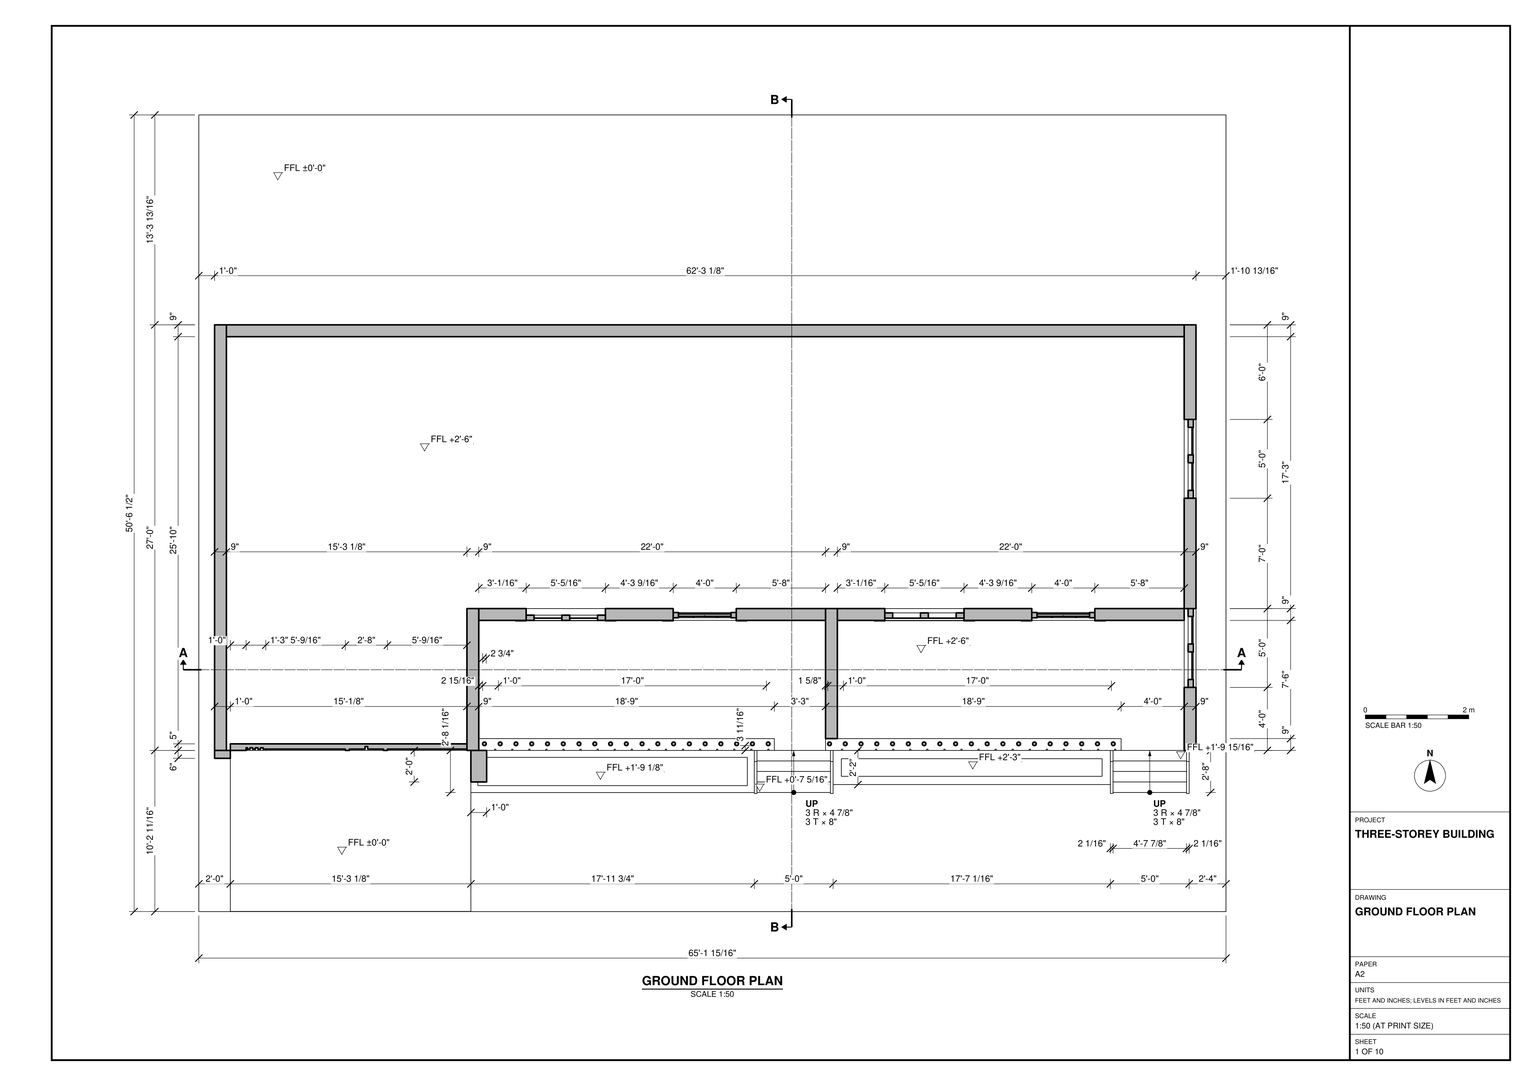
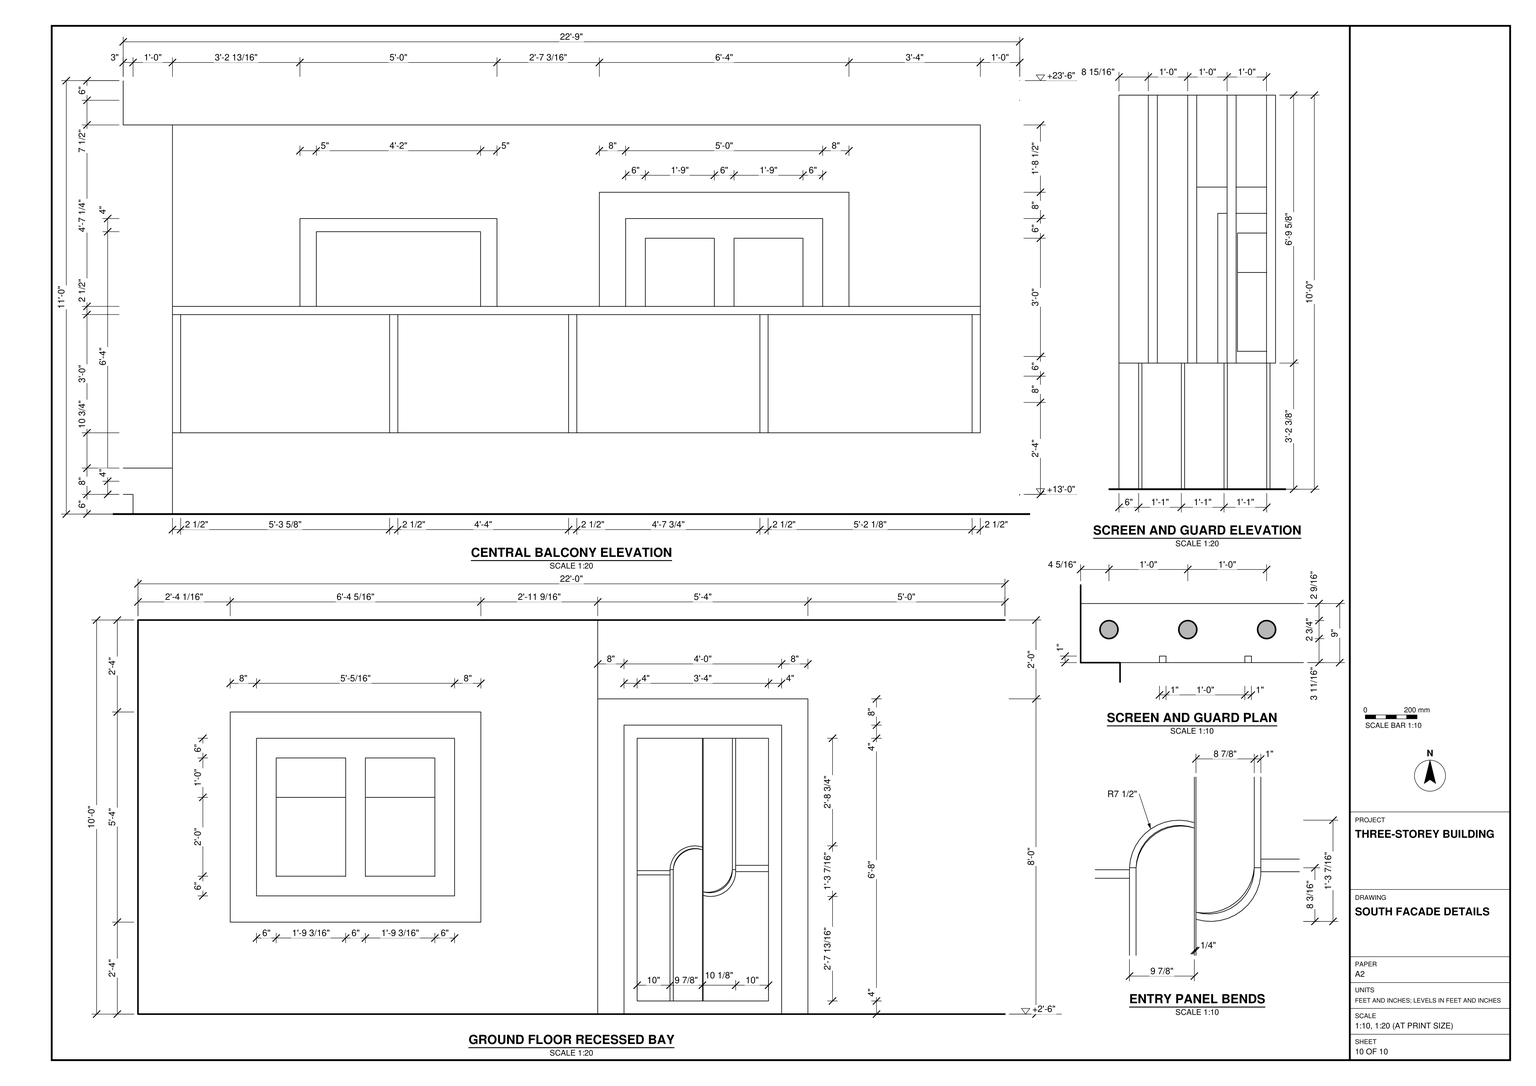
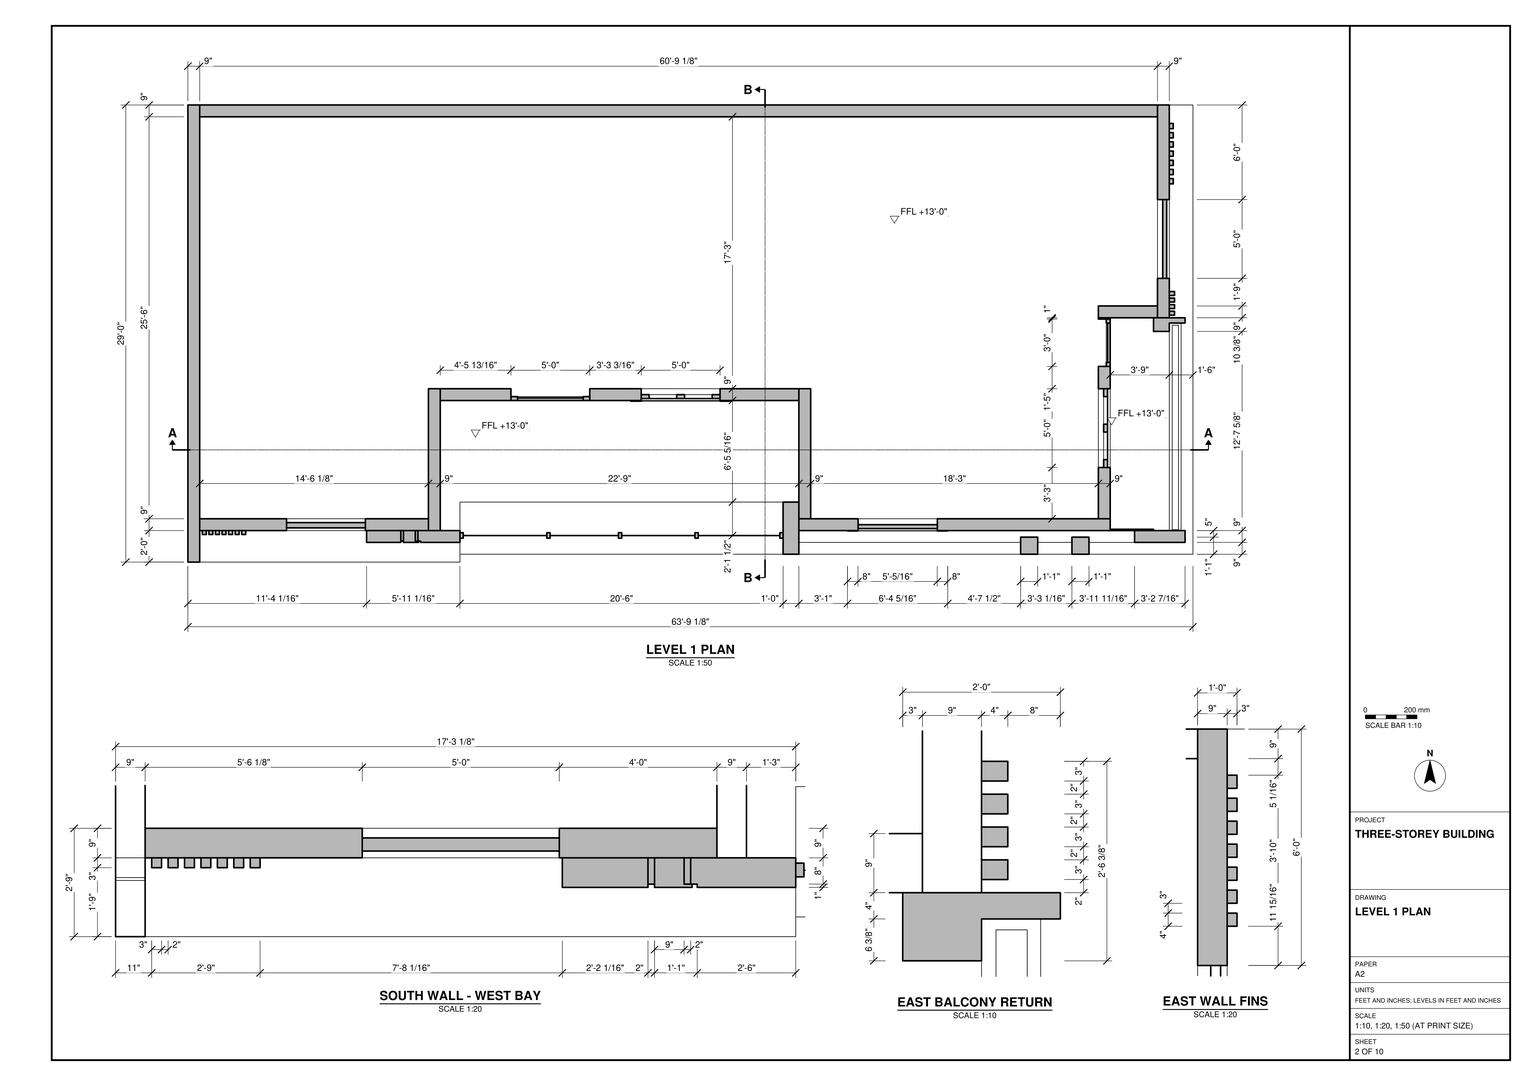
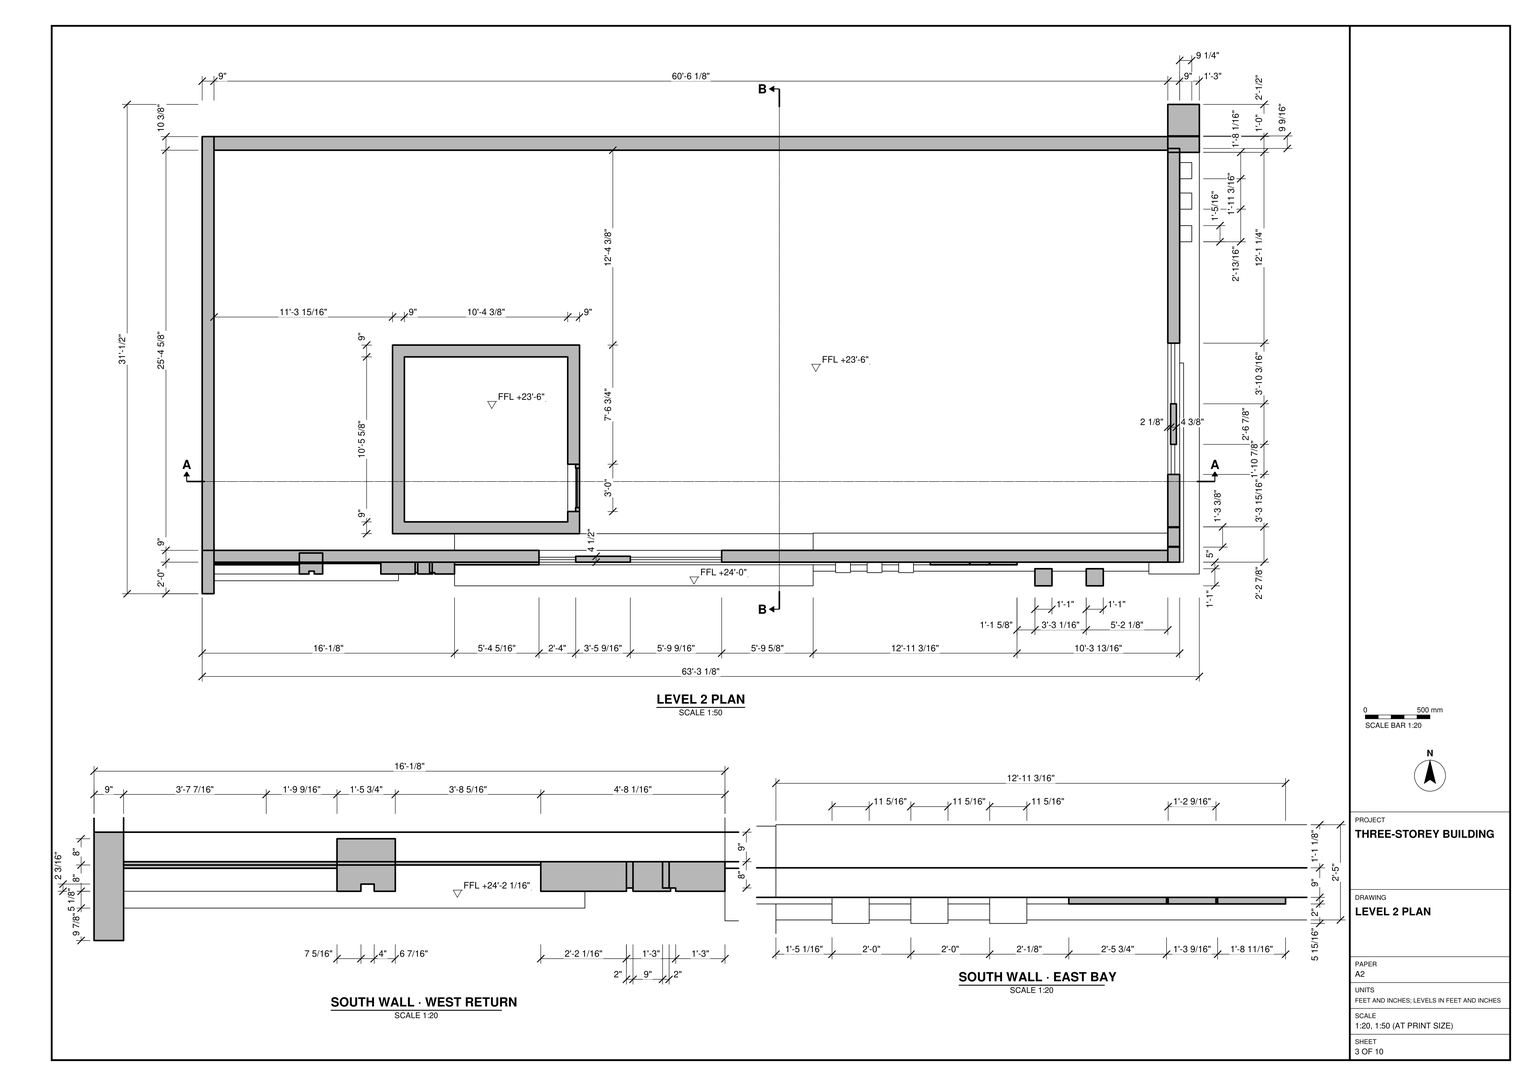
Build the three-storey building in SketchUp from task_files/diagram_01.pdf. Work in feet and inches. The overall model, including its base, is 65'-3 1/8" along x, 50'-6 1/2" along y and 35'-1 7/8" high. Use the levels ±0'-0", +13'-0" and +23'-6". Distinguish the ground datum from the raised ground-floor surface marked +2'-6".

Lay out each storey from its own plan. Model the walls at the thicknesses drawn, including the 9" perimeter walls, and follow the slab and roof outlines. On the south side, form the two recessed ground-floor bays with their dividing wall, framed windows, inset entry doors and short approach steps. Use the enlarged entry detail for the opposing bends in the door panels. Above these bays, set back the wall behind the central balcony and carry the guard across its front. Follow the details for the east balcony return, the wall fins and the screen above the guard. Place other openings, stairs, built-in joinery and main furniture where the sheets indicate them.

Keep walls, slabs, roof elements and each furniture or joinery piece in separate groups or components. Use components for repeated parts such as matching window units and fins. Decor and loose items, where shown, may be any suitable library components. Save one SketchUp model as output_files/three_storey_building_with_recessed_bays_and_balconies.skp.

# SketchUp Ruby script. Lengths in inches.
U = 1.inch
M = Sketchup.active_model
def pt(a) = Geom::Point3d.new(a.map { |v| v * U })
def face(e, loops, mat)
  f = e.add_face(loops[0].map { |a| pt(a) })
  loops[1..].each { |l| e.add_face(l.map { |a| pt(a) }).erase! }
  f.material = f.back_material = mat if mat
  f
end
# faces: each face lists its corners as indices into pts; further lists are holes
def faces(e, pts, list, mat = nil) = list.each { |f| face(e, (f[0].is_a?(Array) ? f : [f]).map { |l| l.map { |i| pts[i] } }, mat) }
# xy, xz, yz: faces in a plane at the given z, y or x. An outline is a flat list of corners, or four numbers for a rectangle; further outlines are holes
def ring(l) = l.size == 4 ? [[l[0], l[1]], [l[2], l[1]], [l[2], l[3]], [l[0], l[3]]] : l.each_slice(2).to_a
def flat(e, list, mat, &to3) = list.each { |f| face(e, (f[0].is_a?(Array) ? f : [f]).map { |l| ring(l).map { |u, v| to3.(u, v) } }, mat) }
def xy(e, z, list, mat = nil) = flat(e, list, mat) { |x, y| [x, y, z] }
def xz(e, y, list, mat = nil) = flat(e, list, mat) { |x, z| [x, y, z] }
def yz(e, x, list, mat = nil) = flat(e, list, mat) { |y, z| [x, y, z] }
def lines(e, pts, list) = list.each { |a, b| e.add_line(pt(pts[a]), pt(pts[b])) }
# prism: a flat outline (further loops are holes) pulled along v
def prism(e, loops, v, mat = nil)
  f = face(e, loops, mat); d = Geom::Vector3d.new(v.map { |x| x * U })
  f.pushpull(f.normal.samedirection?(d) ? d.length : -d.length)
end
def box(e, o, s, mat = nil) = prism(e, [[o, [o[0] + s[0], o[1], o[2]], [o[0] + s[0], o[1] + s[1], o[2]], [o[0], o[1] + s[1], o[2]]]], [0, 0, s[2]], mat)
def at(x, y, z, deg = 0) = Geom::Transformation.translation(pt([x, y, z])) * Geom::Transformation.rotation(ORIGIN, Z_AXIS, deg.degrees)
def axes(o, x, y, z) = Geom::Transformation.new([*x, 0, *y, 0, *z, 0, *pt(o).to_a, 1])
def part(name) = M.definitions.add(name)
# library, detail: a bought-in or finely detailed component or shape, given as its bounding box
def library(name, o, s) = part(name).tap { |d| box(d.entities, o, s) }
def detail(e, o, s) = box(e.add_group.entities, o, s)
def put(e, d, t, mat = nil) = e.add_instance(d, t).tap { |i| i.material = mat if mat }
def group(e, t, mat = nil) = e.add_group.tap { |g| g.transformation = t; g.material = mat if mat }.entities
root = M.entities
M.materials.add("[Color C01]").color = [209, 187, 166]
M.materials.add("[Color J01]").color = [112, 99, 124]
M.materials.add("[Color L11]").color = [109, 70, 75]
M.materials.add("[Color M00]").color = [255, 255, 255]
M.materials.add("[Color M02]").color = [198, 198, 198]
M.materials.add("[Color M05]").color = [114, 114, 114]
M.materials.add("[Color M07]").color = [58, 58, 58]
M.materials.add("[Color M08]").color = [30, 30, 30]
M.materials.add("[Color M09]").color = [0, 0, 0]
M.materials.add("[Concrete Stamped Ashlar]").color = [128, 71, 66]
M.materials.add("[Field Rectangle Tile]").color = [196, 189, 179]
M.materials.add("[Grass Dark Green]").color = [106, 157, 55]
M.materials.add("[Translucent Glass Gray]").color = [128, 128, 128]
M.materials["[Translucent Glass Gray]"].alpha = 0.5
M.materials.add("[Wood Bamboo]").color = [177, 105, 43]
M.materials.add("[Wood Cherry Original]").color = [152, 86, 42]
M.materials.add("[Wood Veneer 01]").color = [48, 28, 14]
c1 = part("Group\#20")
xz(c1.entities,0,[[0,0,21.16,36]])
c2 = part("Group\#21")
xz(c2.entities,0,[[0,0,21.16,36]])
c3 = part("Group\#41")
prism(c3.entities,[[[225,0,0],[221,0,0],[221,1,0],[220,1,0],[220,0,0],[208,0,0],[208,1,0],[207,1,0],[207,0,0],[195,0,0],[195,1,0],[194,1,0],[194,0,0],[182,0,0],[182,1,0],[181,1,0],[181,0,0],[169,0,0],[169,1,0],[168,1,0],[168,0,0],[156,0,0],[156,1,0],[155,1,0],[155,0,0],[143,0,0],[143,1,0],[142,1,0],[142,0,0],[130,0,0],[130,1,0],[129,1,0],[129,0,0],[117,0,0],[117,1,0],[116,1,0],[116,0,0],[104,0,0],[104,1,0],[103,1,0],[103,0,0],[91,0,0],[91,1,0],[90,1,0],[90,0,0],[78,0,0],[78,1,0],[77,1,0],[77,0,0],[65,0,0],[65,1,0],[64,1,0],[64,0,0],[52,0,0],[52,1,0],[51,1,0],[51,0,0],[39,0,0],[39,1,0],[38,1,0],[38,0,0],[26,0,0],[26,1,0],[25,1,0],[25,0,0],[13,0,0],[13,1,0],[12,1,0],[12,0,0],[0,0,0],[0,9,0],[225,9,0]]],[0,0,38.4])
c4 = library("Group\#42",[0,0,0],[60,32.82,59.54])
c5 = library("Group\#43",[0,0,0],[60,32.82,59.54])
c6 = part("Group\#52")
box(c6.entities,[0,0,0],[3,4,120])
c7 = part("Group\#127")
prism(c7.entities,[[[76.32,0.3,0],[0,0.3,0],[0,0.3,64],[76.32,0.3,64]],[[8,0.3,56],[8,0.3,8],[68.32,0.3,8],[68.32,0.3,56]]],[0,-0.3,0])
c8 = part("Group\#15")
prism(c8.entities,[[[64,0.3,0],[56,0.3,0],[56,0.3,88],[8,0.3,88],[8,0.3,0],[0,0.3,0],[0,0.3,96],[64,0.3,96]]],[0,-0.3,0])
p = [[8,0.3,0],[56,0.3,0]]
lines(c8.entities,p,[[0,1]])
c9 = library("Group\#23",[0,0,0],[48,4,88])
c10 = part("Group\#19")
prism(c10.entities,[[[0,0,48],[0,0,0],[60.32,0,0],[60.32,0,48]],[[33.16,0,42],[54.32,0,42],[54.32,0,6],[33.16,0,6]],[[27.16,0,42],[27.16,0,6],[6,0,6],[6,0,42]]],[0,4,0])
c11 = part("Group\#11")
prism(c11.entities,[[[0,78,4.5],[0,78,0.3],[0,70,0.3],[0,70,0],[0,68,0],[0,68,0.3],[0,60,0.3],[0,60,0],[0,58,0],[0,58,0.3],[0,50,0.3],[0,50,0],[0,48,0],[0,48,0.3],[0,40,0.3],[0,40,0],[0,38,0],[0,38,0.3],[0,30,0.3],[0,30,0],[0,28,0],[0,28,0.3],[0,20,0.3],[0,20,0],[0,18,0],[0,18,0.3],[0,10,0.3],[0,10,0],[0,8,0],[0,8,0.3],[0,0,0.3],[0,0,4.5],[0,8,4.5],[0,8,4],[0,10,4],[0,10,4.5],[0,18,4.5],[0,18,4],[0,20,4],[0,20,4.5],[0,28,4.5],[0,28,4],[0,30,4],[0,30,4.5],[0,38,4.5],[0,38,4],[0,40,4],[0,40,4.5],[0,48,4.5],[0,48,4],[0,50,4],[0,50,4.5],[0,58,4.5],[0,58,4],[0,60,4],[0,60,4.5],[0,68,4.5],[0,68,4],[0,70,4],[0,70,4.5]]],[30,0,0])
c12 = part("Group\#74")
box(c12.entities,[0,0,0],[4,3,120])
c13 = part("Group\#75")
box(c13.entities,[0,0,0],[4.75,2.9375,30])
c14 = part("Group\#83")
box(c14.entities,[0,0,0],[9.25,12.3125,20.4375])
c15 = part("Group\#84")
prism(c15.entities,[[[2.57,99.9375,2.0625],[2.7,99.9375,1.73],[2.75,99.9375,1.375],[2.7,99.9375,1.02],[2.57,99.9375,0.6875],[2.35,99.9375,0.4],[2.0625,99.9375,0.18],[1.73,99.9375,0.05],[1.375,99.9375,0],[1.02,99.9375,0.05],[0.6875,99.9375,0.18],[0.4,99.9375,0.4],[0.18,99.9375,0.6875],[0.05,99.9375,1.02],[0,99.9375,1.375],[0.05,99.9375,1.73],[0.18,99.9375,2.0625],[0.4,99.9375,2.35],[0.6875,99.9375,2.57],[1.02,99.9375,2.7],[1.375,99.9375,2.75],[1.73,99.9375,2.7],[2.0625,99.9375,2.57],[2.35,99.9375,2.35]]],[0,-99.9375,0])
c16 = library("Group\#86",[0,-2,0],[180.12,5,114])
c17 = part("Group\#91")
box(c17.entities,[0,0,0],[3,3,112])
c18 = part("Group\#94")
box(c18.entities,[0,0.625,-26.4],[12.98,13,201.25])
c19 = part("Group\#99")
box(c19.entities,[0,0,0],[2.5,4.1875,36])
c20 = part("Group\#110")
prism(c20.entities,[[[0,1.84,0.69],[0,1.75,0.47],[0,1.6,0.27],[0,1.41,0.125],[0,1.18,0.03],[0,0.9375,0],[0,0.69,0.03],[0,0.47,0.125],[0,0.27,0.27],[0,0.125,0.47],[0,0.03,0.69],[0,0,0.9375],[0,0.03,1.18],[0,0.125,1.41],[0,0.27,1.6],[0,0.47,1.75],[0,0.69,1.84],[0,0.9375,1.875],[0,1.18,1.84],[0,1.41,1.75],[0,1.6,1.6],[0,1.75,1.41],[0,1.84,1.18],[0,1.875,0.9375]]],[139.0625,0,0])
c21 = part("Group\#113")
prism(c21.entities,[[[64.98,1.52,0.41],[64.98,1.6,0.6],[64.98,1.625,0.8125],[64.98,1.6,1.02],[64.98,1.52,1.22],[64.98,1.39,1.39],[64.98,1.22,1.52],[64.98,1.02,1.6],[64.98,0.8125,1.625],[64.98,0.6,1.6],[64.98,0.41,1.52],[64.98,0.24,1.39],[64.98,0.11,1.22],[64.98,0.03,1.02],[64.98,0,0.8125],[64.98,0.03,0.6],[64.98,0.11,0.41],[64.98,0.24,0.24],[64.98,0.41,0.11],[64.98,0.6,0.03],[64.98,0.8125,0],[64.98,1.02,0.03],[64.98,1.22,0.11],[64.98,1.39,0.24]]],[-64.98,0,0])
c22 = part("Group\#129")
prism(c22.entities,[[[0.18,2.0625,0],[0.4,2.35,0],[0.6875,2.57,0],[1.02,2.7,0],[1.375,2.75,0],[1.73,2.7,0],[2.0625,2.57,0],[2.35,2.35,0],[2.57,2.0625,0],[2.7,1.73,0],[2.75,1.375,0],[2.7,1.02,0],[2.57,0.6875,0],[2.35,0.4,0],[2.0625,0.18,0],[1.73,0.05,0],[1.375,0,0],[1.02,0.05,0],[0.6875,0.18,0],[0.4,0.4,0],[0.18,0.6875,0],[0.05,1.02,0],[0,1.375,0],[0.05,1.73,0]]],[0,0,81.6])
xz(root,90.68,[[693.92,31.32,695.97,67.32]],"[Color M08]")
p = [[756.11,274.31,312],[756.11,434.68,312],[756.11,434.68,360]]
lines(root,p,[[0,1],[1,2]])
g1 = group(root,at(120,44.5,0))
box(g1,[-120,-44.5,0],[781.9375,606.5,24])
g2 = group(root,at(150.11,86.68,6))
box(g2,[-138.11,36,18],[738.11,324,30])
put(root,c1,at(282.36,223.38,84),"[Translucent Glass Gray]")
put(root,c2,at(255.2,223.38,84),"[Translucent Glass Gray]")
put(root,c3,at(477.11,122.68,54),"[Concrete Stamped Ashlar]")
put(root,c4,at(693.92,89.86,24))
put(root,c5,at(422.86,89.86,24))
put(root,c3,at(213.12,122.68,54),"[Concrete Stamped Ashlar]")
g3 = group(root,at(12,122.68,54))
box(g3,[0,0,0],[9,324,120])
g4 = group(root,at(207.12,110.68,24))
xy(g4,0,[[0,-12,12,12]])
xy(g4,156,[[-195.12,-12,-195.12,336,-186.12,336,-186.12,12,0,12,0,-12]])
xy(g4,164,[[-186.12,-12,12,12]])
xy(g4,282,[[-195.12,21,-186.12,336]])
xy(g4,388.875,[[-186.12,-12,-65.99,21]])
xy(g4,397.875,[[-195.12,-12,-65.99,21]])
xz(g4,-12,[[0,0,12,0,12,164,-186.12,164,-186.12,388.875,-65.99,388.875,-65.99,397.875,-195.12,397.875,-195.12,156,0,156]])
xz(g4,12,[[0,0,0,156,-186.12,156,-186.12,164,12,164,12,0]])
xz(g4,21,[[-195.12,282,-195.12,397.875,-65.99,397.875,-65.99,388.875,-186.12,388.875,-186.12,282]])
xz(g4,336,[[-195.12,156,-186.12,282]])
yz(g4,-195.12,[[-12,156,-12,397.875,21,397.875,21,282,336,282,336,156]])
yz(g4,-186.12,[[12,156,336,164],[-12,164,336,164,336,282,21,282,21,388.875,-12,388.875]])
yz(g4,-65.99,[[-12,388.875,21,397.875]])
yz(g4,0,[[-12,0,12,156]])
yz(g4,12,[[-12,0,12,164]])
g5 = group(root,at(12,116.68,24),"[Color J01]")
prism(g5,[[[0,0,0],[12,0,0],[12,0,144],[195.12,0,144],[195.12,0,156],[0,0,156]]],[0,6,0])
put(root,c6,at(759.11,428.64,180),"[Color L11]")
put(root,c6,at(759.11,421.64,180),"[Color L11]")
put(root,c6,at(759.11,414.64,180),"[Color L11]")
put(root,c6,at(759.11,407.64,180),"[Color L11]")
put(root,c6,at(759.11,400.64,180),"[Color L11]")
put(root,c6,at(759.11,393.64,180),"[Color L11]")
put(root,c6,at(759.11,386.64,180),"[Color L11]")
put(root,c1,at(555.36,223.38,96),"[Translucent Glass Gray]")
g6 = group(root,at(757.11,347.68,228),"[Translucent Glass Gray]")
yz(g6,0,[[0,0,21,36]])
g7 = group(root,at(754.11,314.68,222),"[Color M07]")
prism(g7,[[[3,60,48],[3,0,48],[3,0,0],[3,60,0]],[[3,33,6],[3,33,42],[3,54,42],[3,54,6]],[[3,6,42],[3,27,42],[3,27,6],[3,6,6]]],[-3,0,0])
g8 = group(root,at(756.11,347.68,96),"[Translucent Glass Gray]")
yz(g8,0,[[0,0,21,36]])
g9 = group(root,at(69.12,437.68,54))
box(g9,[-48.12,0,0],[729.11,9,120])
g10 = group(root,at(367.5,221.68,54),"[Color C01]")
xy(g10,0,[[118.62,0,266.61,9],[314.61,0,382.61,9]])
xy(g10,36,[[154.7,0,215.02,9]])
xy(g10,84,[[154.7,0,215.02,9]])
xy(g10,88,[[266.61,0,314.61,9]])
xy(g10,120,[[118.62,0,382.61,9]])
xz(g10,0,[[258.61,0,266.61,0,266.61,88,314.61,88,314.61,0,382.61,0,382.61,120,258.61,120]])
xz(g10,0,[[[118.62,0,258.61,120],[154.7,36,215.02,84]]],"[Field Rectangle Tile]")
xz(g10,9,[[[118.62,0,118.62,120,382.61,120,382.61,0,314.61,0,314.61,88,266.61,88,266.61,0],[154.7,36,215.02,84]]])
yz(g10,118.62,[[0,0,9,120]])
yz(g10,154.7,[[0,36,9,84]])
yz(g10,215.02,[[0,36,9,84]])
yz(g10,266.61,[[0,0,9,88]])
yz(g10,314.61,[[0,0,9,88]])
yz(g10,382.61,[[0,0,9,120]])
put(root,c7,at(514.2,221.38,82),"[Wood Veneer 01]")
put(root,c8,at(626.11,221.38,54),"[Wood Veneer 01]")
g11 = group(root,at(757.11,320.68,228),"[Translucent Glass Gray]")
yz(g11,0,[[0,0,21,36]])
g12 = group(root,at(756.11,320.68,96),"[Translucent Glass Gray]")
yz(g12,0,[[0,0,21,36]])
put(root,c9,at(634.11,223.68,54))
g13 = group(root,at(750.11,284.68,180),"[Color C01]")
prism(g13,[[[0,162,0],[0,0,0],[0,0,120],[0,162,120]],[[0,30,90],[0,30,42],[0,90,42],[0,90,90]]],[9,0,0])
g14 = group(root,at(204.12,122.68,174))
xy(g14,0,[[273,-18,273,0,-192.12,0,-192.12,324,572.99,324,572.99,-18]])
xy(g14,6,[[273,-18,572.99,-18,572.99,324,-192.12,324,-192.12,0,273,0]])
xz(g14,-18,[[273,0,572.99,6]],"[Color L11]")
xz(g14,0,[[-192.12,0,273,6]])
xz(g14,324,[[-192.12,0,572.99,6]])
yz(g14,-192.12,[[0,0,324,6]])
yz(g14,273,[[-18,0,0,6]])
yz(g14,572.99,[[-18,0,324,6]],"[Color L11]")
p = [[273,9,0],[273,9,6],[271.2,0,0]]
lines(g14,p,[[0,1],[1,2]])
put(root,c7,at(241.2,221.38,82),"[Wood Veneer 01]")
put(root,c9,at(361.11,223.68,54))
put(root,c8,at(353.11,221.38,54),"[Wood Veneer 01]")
g15 = group(root,at(94.5,221.68,54),"[Color C01]")
xy(g15,0,[[118.62,0,266.61,9],[314.61,0,382.61,9]],"[Field Rectangle Tile]")
xy(g15,36,[[154.7,0,215.02,9]],"[Field Rectangle Tile]")
xy(g15,84,[[154.7,0,215.02,9]],"[Field Rectangle Tile]")
xy(g15,88,[[266.61,0,314.61,9]],"[Field Rectangle Tile]")
xy(g15,120,[[118.62,0,382.61,9]],"[Field Rectangle Tile]")
xz(g15,0,[[258.61,0,266.61,0,266.61,88,314.61,88,314.61,0,382.61,0,382.61,120,258.61,120]])
xz(g15,0,[[[118.62,0,258.61,120],[154.7,36,215.02,84]]],"[Field Rectangle Tile]")
xz(g15,9,[[[118.62,0,118.62,120,382.61,120,382.61,0,314.61,0,314.61,88,266.61,88,266.61,0],[154.7,36,215.02,84]]],"[Field Rectangle Tile]")
yz(g15,118.62,[[0,0,9,120]],"[Field Rectangle Tile]")
yz(g15,154.7,[[0,36,9,84]],"[Field Rectangle Tile]")
yz(g15,215.02,[[0,36,9,84]],"[Field Rectangle Tile]")
yz(g15,266.61,[[0,0,9,88]],"[Field Rectangle Tile]")
yz(g15,314.61,[[0,0,9,88]],"[Field Rectangle Tile]")
yz(g15,382.61,[[0,0,9,120]],"[Field Rectangle Tile]")
g16 = group(root,at(204.12,122.68,54))
xy(g16,0,[[0,0,9,108]])
xy(g16,120,[[0,0,9,108]])
xz(g16,0,[[0,0,9,120]])
xz(g16,108,[[0,0,9,120]])
yz(g16,0,[[0,0,108,120]])
yz(g16,9,[[0,0,108,120]],"[Field Rectangle Tile]")
put(root,c10,at(249.2,221.68,90),"[Color M07]")
g17 = group(root,at(477.11,110.68,54))
xy(g17,0,[[0,21,9,120]])
xy(g17,120,[[0,21,9,120]])
xz(g17,21,[[0,0,9,120]])
xz(g17,120,[[0,0,9,120]])
yz(g17,0,[[21,0,120,120]])
yz(g17,9,[[21,0,120,120]],"[Field Rectangle Tile]")
put(root,c11,axes([759.11,305.68,138],[0.8,0,0],[0,1,0],[0,0,1]),"[Color L11]")
g18 = group(root,at(753.11,314.68,90),"[Color M07]")
prism(g18,[[[0,0,0],[0,0,48],[0,60,48],[0,60,0]],[[0,33,42],[0,33,6],[0,54,6],[0,54,42]],[[0,27,42],[0,6,42],[0,6,6],[0,27,6]]],[4,0,0])
g19 = group(root,at(750.11,98.68,18),"[Color C01]")
prism(g19,[[[9,24,6],[9,348,6],[9,348,156],[9,24,156]],[[9,132,120],[9,132,72],[9,72,72],[9,72,120]],[[9,216,72],[9,216,120],[9,276,120],[9,276,72]]],[-9,0,0])
put(root,c2,at(528.2,223.38,96),"[Translucent Glass Gray]")
put(root,c11,axes([759.11,305.68,269.97],[0.8,0,0],[0,1,0],[0,0,1]),"[Color L11]")
put(root,c10,at(522.2,223.38,90),"[Color M07]")
g20 = group(root,at(753.11,170.68,90),"[Color M07]")
prism(g20,[[[0,60,48],[0,60,0],[0,0,0],[0,0,48]],[[0,33,42],[0,33,6],[0,54,6],[0,54,42]],[[0,27,42],[0,6,42],[0,6,6],[0,27,6]]],[4,0,0])
g21 = group(root,at(756.11,176.68,96),"[Translucent Glass Gray]")
yz(g21,0,[[0,0,21,36]])
g22 = group(root,at(756.11,203.68,96),"[Translucent Glass Gray]")
yz(g22,0,[[0,0,21,36]])
g23 = group(root,at(759.11,161.68,138),"[Color L11]")
prism(g23,[[[0,78,4.5],[0,78,0.3],[0,70,0.3],[0,70,0],[0,68,0],[0,68,0.3],[0,60,0.3],[0,60,0],[0,58,0],[0,58,0.3],[0,50,0.3],[0,50,0],[0,48,0],[0,48,0.3],[0,40,0.3],[0,40,0],[0,38,0],[0,38,0.3],[0,30,0.3],[0,30,0],[0,28,0],[0,28,0.3],[0,20,0.3],[0,20,0],[0,18,0],[0,18,0.3],[0,10,0.3],[0,10,0],[0,8,0],[0,8,0.3],[0,0,0.3],[0,0,4.5],[0,8,4.5],[0,8,4],[0,10,4],[0,10,4.5],[0,18,4.5],[0,18,4],[0,20,4],[0,20,4.5],[0,28,4.5],[0,28,4],[0,30,4],[0,30,4.5],[0,38,4.5],[0,38,4],[0,40,4],[0,40,4.5],[0,48,4.5],[0,48,4],[0,50,4],[0,50,4.5],[0,58,4.5],[0,58,4],[0,60,4],[0,60,4.5],[0,68,4.5],[0,68,4],[0,70,4],[0,70,4.5]]],[24,0,0])
g24 = group(root,at(705.11,284.68,180))
box(g24,[0,0,0],[45,9,120])
g25 = group(root,at(705.11,176.68,180),"[Color C01]")
prism(g25,[[[0,71,0],[0,-45,0],[0,-45,120],[0,108,120],[0,108,0],[0,107,0],[0,107,89],[0,71,89]],[[0,-6,89],[0,-6,36],[0,54,36],[0,54,89]]],[9,0,0])
g26 = group(root,at(711.11,247.68,180),"[Wood Cherry Original]")
prism(g26,[[[3,36,0],[3,36,89],[3,0,89],[3,0,0]],[[3,33,3],[3,3,3],[3,3,86],[3,33,86]]],[-3,0,0])
g27 = group(root,at(712.11,250.68,183),"[Wood Cherry Original]")
box(g27,[0,0,0],[2,30,83])
g28 = group(root,at(477.11,122.68,180),"[Color J01]")
prism(g28,[[[237,9,0],[0,9,0],[0,9,120],[237,9,120]],[[105.41,9,90],[45.09,9,90],[45.09,9,42],[105.41,9,42]]],[0,-9,0])
g29 = group(root,at(709.11,170.68,216),"[Color M07]")
prism(g29,[[[0,0,0],[0,0,53],[0,60,53],[0,60,0]],[[0,33,47],[0,33,6],[0,54,6],[0,54,47]],[[0,27,47],[0,6,47],[0,6,6],[0,27,6]]],[3,0,0])
g30 = group(root,at(712.11,203.68,222),"[Translucent Glass Gray]")
yz(g30,0,[[0,0,21,41]])
g31 = group(root,at(712.11,176.68,222),"[Translucent Glass Gray]")
yz(g31,0,[[0,0,21,41]])
g32 = group(root,at(477.11,131.68,180))
box(g32,[0,0,0],[9,99,120])
g33 = group(root,at(29.87,221.68,180),"[Color C01]")
prism(g33,[[[447.24,9,0],[288.0625,9,0],[288.0625,9,84],[228.0625,9,84],[228.0625,9,0],[174.25,9,0],[174.25,9,120],[447.24,9,120]],[[387.24,9,84],[327.24,9,84],[327.24,9,36],[387.24,9,36]]],[0,-9,0])
g34 = group(root,at(195.12,122.68,180),"[Color C01]")
box(g34,[0,0,0],[9,108,120])
g35 = group(root,at(257.93,221.68,180))
g36 = group(g35,at(5,0,4),"[Wood Bamboo]")
box(g36,[0,0,0],[50,2,76])
g37 = group(g35,at(0,0,0),"[Wood Veneer 01]")
prism(g37,[[[60,3,84],[60,3,0],[0,3,0],[0,3,84]],[[55,3,4],[55,3,80],[5,3,80],[5,3,4]]],[0,-3,0])
g38 = group(root,at(357.11,223.18,216),"[Color M07]")
prism(g38,[[[0,3,48],[60,3,48],[60,3,0],[0,3,0]],[[27,3,6],[27,3,42],[6,3,42],[6,3,6]],[[54,3,42],[33,3,42],[33,3,6],[54,3,6]]],[0,-3,0])
g39 = group(root,at(390.11,223.18,222),"[Translucent Glass Gray]")
xz(g39,0,[[0,0,21,36]])
g40 = group(root,at(363.11,223.18,222),"[Translucent Glass Gray]")
xz(g40,0,[[0,0,21,36]])
g41 = group(root,at(349.11,221.18,208),"[Color L11]")
prism(g41,[[[0,0,0],[76,0,0],[76,0,64],[0,0,64]],[[8,0,56],[68,0,56],[68,0,8],[8,0,8]]],[0,0.5,0])
g42 = group(root,at(195.12,110.68,174))
xy(g42,0,[[24,-6,282,33.6875]])
xy(g42,6,[[282,3,575.99,12],[563.99,12,572.99,170],[551.99,163.625,551.99,174,575.99,174,575.99,170,563.99,170,563.99,163.625]])
xy(g42,18,[[563.99,12,572.99,170]])
xy(g42,24.75,[[24,-6,270,33.6875]])
xy(g42,44.375,[[282,3,537.56,12]])
xy(g42,102,[[563.99,12,575.99,170]])
xy(g42,118.5,[[9,-6,270,33.6875]],"[Color L11]")
xy(g42,126,[[551.99,174,575.99,336],[551.99,336,574.99,336.5],[551.99,336.5,575.99,360.5]])
xy(g42,138,[[9,-6,282,33.6875],[537.56,3,575.99,3,575.99,324,551.99,324,551.99,163.625,563.99,163.625,563.99,12,537.56,12]])
xy(g42,174,[[551.99,336,574.99,336.5]])
xy(g42,186,[[551.99,230.6875,575.99,324]])
xy(g42,195.25,[[551.99,230.6875,575.99,336],[551.99,336.5,575.99,360.5]])
xz(g42,-6,[[24,0,282,0,282,138,9,138,9,118.5,270,118.5,270,24.75,24,24.75]],"[Color L11]")
xz(g42,3,[[282,6,575.99,6,575.99,138,537.56,138,537.56,44.375,282,44.375]])
xz(g42,12,[[282,6,282,44.375,537.56,44.375,537.56,138,563.99,138,563.99,102,575.99,102,575.99,6,572.99,6,572.99,18,563.99,18,563.99,6],[563.99,6,572.99,18]])
xz(g42,33.6875,[[24,0,24,24.75,270,24.75,270,118.5,9,118.5,9,138,282,138,282,0]])
xz(g42,163.625,[[551.99,6,563.99,138]])
xz(g42,170,[[563.99,6,572.99,18],[572.99,6,575.99,6,575.99,102,563.99,102,563.99,18,572.99,18]])
xz(g42,174,[[551.99,6,575.99,126]])
xz(g42,230.6875,[[551.99,186,575.99,195.25]])
xz(g42,324,[[551.99,138,575.99,186]])
xz(g42,336,[[551.99,126,574.99,174],[574.99,126,575.99,174],[551.99,174,575.99,195.25]])
xz(g42,336.5,[[551.99,126,574.99,174],[574.99,126,575.99,174],[551.99,174,575.99,195.25]])
xz(g42,360.5,[[551.99,126,575.99,195.25]])
yz(g42,9,[[-6,118.5,33.6875,138]],"[Color L11]")
yz(g42,24,[[-6,0,33.6875,24.75]],"[Color L11]")
yz(g42,270,[[-6,24.75,33.6875,118.5]],"[Color L11]")
yz(g42,282,[[3,6,12,44.375],[12,6,33.6875,48]])
yz(g42,282,[[-6,0,33.6875,0,33.6875,6,3,6,3,44.375,12,44.375,12,48,33.6875,48,33.6875,138,-6,138]],"[Color L11]")
yz(g42,537.56,[[3,44.375,12,138]])
yz(g42,551.99,[[163.625,6,163.625,138,324,138,324,186,230.6875,186,230.6875,195.25,336,195.25,336,126,174,126,174,6],[336,126,336.5,174],[336.5,126,360.5,195.25]])
yz(g42,563.99,[[12,6,163.625,18],[163.625,6,170,18],[163.625,18,170,102],[12,102,163.625,138]])
yz(g42,572.99,[[12,6,170,18]],"[Color M07]")
yz(g42,574.99,[[336,126,336.5,174]])
yz(g42,575.99,[[3,6,12,6,12,102,170,102,170,6,174,6,174,126,336,126,336,195.25,230.6875,195.25,230.6875,186,324,186,324,138,3,138],[336.5,126,360.5,195.25]])
put(root,c12,at(759.11,286.68,180))
put(root,c12,at(759.11,291.68,180))
put(root,c12,at(759.11,296.68,180))
put(root,c12,at(759.11,301.68,180))
put(root,c13,at(761.3125,276.08,192),"[Color M09]")
put(root,c13,at(761.3125,217.77,192),"[Color M09]")
put(root,c13,at(761.3125,167.02,192),"[Color M09]")
put(root,c13,at(761.3125,123.4,192),"[Color M09]")
g43 = group(root,at(764.0625,220.71,192),"[Translucent Glass Gray]")
yz(g43,0,[[0,0,55.375,30]])
g44 = group(root,at(764.0625,169.96,192),"[Translucent Glass Gray]")
yz(g44,0,[[0,0,47.8125,30]])
g45 = group(root,at(764.0625,126.33,192),"[Translucent Glass Gray]")
yz(g45,0,[[0,0,40.6875,30]])
g46 = group(root,at(761.3125,123.4,222),"[Color M09]")
box(g46,[0,0,0],[4.75,155.625,1.4375])
g47 = group(root,at(12,437.68,180))
box(g47,[9,0,0],[729.11,9,120])
g48 = group(root,at(195.12,122.68,300))
prism(g48,[[[-174.12,0,0],[-174.12,324,0],[551.99,324,0],[551.99,151.625,0],[563.99,151.625,0],[563.99,0,0]]],[0,0,6])
g49 = group(root,at(747.11,122.68,306),"[Color C01]")
xy(g49,0,[[0,0,9,11.48],[0,11.48,9,11.98],[0,11.98,9,26.375],[0,26.375,9,26.875],[0,26.875,9,314.96]])
xy(g49,10.7,[[0,66.8,9,166.74]])
xy(g49,52.14,[[0,66.8,9,93.13]])
xy(g49,63.25,[[0,0,9,11.48],[0,11.48,9,11.98],[0,11.98,9,26.375],[0,26.375,9,26.875],[0,26.875,9,93.13],
  [0,166.74,9,314.96]])
xz(g49,0,[[0,0,9,63.25]])
xz(g49,11.48,[[0,0,9,63.25]])
xz(g49,11.98,[[0,0,9,63.25]])
xz(g49,26.375,[[0,0,9,63.25]])
xz(g49,26.875,[[0,0,9,63.25]])
xz(g49,66.8,[[0,10.7,9,52.14]])
xz(g49,93.13,[[0,52.14,9,63.25]])
xz(g49,166.74,[[0,10.7,9,63.25]])
xz(g49,314.96,[[0,0,9,63.25]])
yz(g49,0,[[0,0,11.48,63.25],[11.48,0,11.98,63.25],[11.98,0,26.375,63.25],[26.375,0,26.875,63.25],[26.875,0,26.875,63.25,93.13,63.25,93.13,52.14,66.8,52.14,66.8,10.7,166.74,10.7,166.74,63.25,314.96,63.25,314.96,0]])
yz(g49,9,[[0,0,11.48,63.25],[11.48,0,11.98,63.25],[11.98,0,26.375,63.25],[26.375,0,26.875,63.25],[26.875,0,314.96,0,314.96,63.25,166.74,63.25,166.74,10.7,66.8,10.7,66.8,52.14,93.13,52.14,93.13,63.25,26.875,63.25]])
put(root,c14,at(756.11,414.6,326.88),"[Color L11]")
put(root,c14,at(756.11,391.41,326.88),"[Color L11]")
put(root,c14,at(756.11,366.6,326.88),"[Color L11]")
put(root,c15,at(749.67,189.48,318.91),"[Color M09]")
put(root,c15,at(749.67,189.48,327.91),"[Color M09]")
put(root,c15,at(749.67,189.48,336.91),"[Color M09]")
put(root,c15,at(749.67,189.48,345.91),"[Color M09]")
put(root,c15,at(749.67,189.48,354.04),"[Color M09]")
put(root,c15,at(749.67,189.48,363.91),"[Color M09]")
g50 = group(root,at(749.23,212.375,316.26),"[Color L11]")
box(g50,[0,0,0],[4.4,30.875,59.74])
put(root,c16,at(24,124.68,54),"[Color M08]")
g51 = group(root,at(21,122.68,180),"[Color C01]")
prism(g51,[[[174.12,9,0],[0,9,0],[0,9,120],[174.12,9,120]],[[126.12,9,44],[126.12,9,92],[66.12,9,92],[66.12,9,44]]],[0,-9,0])
g52 = group(root,at(87.12,124.74,224),"[Color M07]")
prism(g52,[[[0,0,48],[0,0,0],[60,0,0],[60,0,48]],[[27,0,42],[27,0,6],[6,0,6],[6,0,42]],[[33,0,42],[54,0,42],[54,0,6],[33,0,6]]],[0,4,0])
g53 = group(root,at(120.12,124.74,230),"[Translucent Glass Gray]")
xz(g53,0,[[0,0,21,36]])
g54 = group(root,at(93.12,124.74,230),"[Translucent Glass Gray]")
xz(g54,0,[[0,0,21,36]])
g55 = group(root,at(77.77,122.18,272),"[Color L11]")
prism(g55,[[[70.6875,-0.25,4.5],[70.6875,-0.25,0.3],[70,-0.24,0.3],[70,-0.24,0],[68,-0.24,0],[68,-0.24,0.3],[60,-0.21,0.3],[60,-0.21,0],[58,-0.2,0],[58,-0.2,0.3],[50,-0.17,0.3],[50,-0.17,0],[48,-0.17,0],[48,-0.17,0.3],[40,-0.14,0.3],[40,-0.14,0],[38,-0.13,0],[38,-0.13,0.3],[30,-0.1,0.3],[30,-0.1,0],[28,-0.1,0],[28,-0.1,0.3],[20,-0.07,0.3],[20,-0.07,0],[18,-0.0625,0],[18,-0.0625,0.3],[10,-0.03,0.3],[10,-0.03,0],[8,-0.03,0],[8,-0.03,0.3],[0,0,0.3],[0,0,4.5],[8,-0.03,4.5],[8,-0.03,4],[10,-0.03,4],[10,-0.03,4.5],[18,-0.0625,4.5],[18,-0.0625,4],[20,-0.07,4],[20,-0.07,4.5],[28,-0.1,4.5],[28,-0.1,4],[30,-0.1,4],[30,-0.1,4.5],[38,-0.13,4.5],[38,-0.13,4],[40,-0.14,4],[40,-0.14,4.5],[48,-0.17,4.5],[48,-0.17,4],[50,-0.17,4],[50,-0.17,4.5],[58,-0.2,4.5],[58,-0.2,4],[60,-0.21,4],[60,-0.21,4.5],[68,-0.24,4.5],[68,-0.24,4],[70,-0.24,4],[70,-0.24,4.5]]],[-0.08,-24,0])
put(root,c17,at(23,119.68,188),"[Color L11]")
put(root,c17,at(28,119.68,188),"[Color L11]")
put(root,c17,at(33,119.68,188),"[Color L11]")
put(root,c17,at(38,119.68,188),"[Color L11]")
put(root,c17,at(43,119.68,188),"[Color L11]")
put(root,c17,at(48,119.68,188),"[Color L11]")
put(root,c17,at(53,119.68,188),"[Color L11]")
g56 = group(root,at(24,0.12,24),"[Color M00]")
prism(g56,[[[183.12,122.5625,0],[183.12,122.5625,30],[183.12,0,0]]],[-183.12,0,0],"[Color M00]")
g57 = group(root,at(12,115.46,154.17),"[Color M05]")
prism(g57,[[[0,1.22,3.4375],[195.12,0.875,3.4375],[195.12,0,3.4375],[0,0.35,3.4375]]],[0,0,22.39])
put(root,c18,at(684.99,104.06,206.4),"[Color L11]")
g58 = group(root,at(294.56,122.68,306),"[Color C01]")
prism(g58,[[[452.55,0,63.25],[112.91,0,63.25],[112.91,0,14.06],[-26.15,0,14.06],[-26.15,0,51.43],[8.26,0,51.43],[8.26,0,63.25],[-273.56,0,63.25],[-273.56,0,0],[452.55,0,0]]],[0,9,0])
g59 = group(root,at(714.11,122.68,206.4),"[Color C01]")
box(g59,[0,0,0],[33,1,86.04])
put(root,c18,at(645.93,104.06,206.4),"[Color L11]")
g60 = group(root,at(148.03,113.68,188),"[Color J01]")
xy(g60,0,[[0,0,26.08,9],[28.08,0,28.08,9,37.08,9,37.08,1,39.52,1,39.52,0],[41.08,0,41.08,1,39.08,1,39.08,9,71.08,9,71.08,0],[26.08,1,28.08,9],[37.08,1,39.08,9]])
xy(g60,112,[[56.08,0,71.08,9]])
xy(g60,181.25,[[0,0,26.08,9],[28.08,0,39.52,0,39.52,1,37.08,1,37.08,9,28.08,9],[41.08,0,56.08,0,56.08,9,39.08,9,39.08,1,41.08,1],[26.08,1,28.08,9],[37.08,1,39.08,9]])
xz(g60,0,[[0,0,26.08,181.25],[28.08,0,39.52,181.25],[41.08,0,71.08,0,71.08,112,56.08,112,56.08,181.25,41.08,181.25]])
xz(g60,1,[[26.08,0,28.08,181.25],[37.08,0,39.08,181.25],[39.08,0,39.52,181.25],[39.52,0,41.08,181.25]])
xz(g60,9,[[0,0,26.08,181.25],[26.08,0,28.08,181.25],[28.08,0,37.08,181.25],[37.08,0,39.08,181.25],[39.08,0,39.08,181.25,56.08,181.25,56.08,112,71.08,112,71.08,0]])
yz(g60,0,[[0,0,9,181.25]])
yz(g60,26.08,[[0,0,1,181.25],[1,0,9,181.25]])
yz(g60,28.08,[[0,0,1,181.25],[1,0,9,181.25]])
yz(g60,37.08,[[1,0,9,181.25]])
yz(g60,39.08,[[1,0,9,181.25]])
yz(g60,39.52,[[0,0,1,181.25]])
yz(g60,41.08,[[0,0,1,181.25]])
yz(g60,56.08,[[0,112,9,181.25]])
yz(g60,71.08,[[0,0,9,112]])
put(root,c19,at(219.12,116.89,198.75),"[Color M09]")
put(root,c19,at(285.24,116.89,198.75),"[Color M09]")
put(root,c19,at(339.74,116.89,198.75),"[Color M09]")
put(root,c19,at(397.99,116.89,198.75),"[Color M09]")
put(root,c19,at(462.61,116.89,198.75),"[Color M09]")
g61 = group(root,at(400.49,118.89,198.75),"[Translucent Glass Gray]")
xz(g61,0,[[0,0,62.12,36]])
g62 = group(root,at(342.24,118.89,198.75),"[Translucent Glass Gray]")
xz(g62,0,[[0,0,55.75,36]])
g63 = group(root,at(287.74,118.89,198.75),"[Translucent Glass Gray]")
xz(g63,0,[[0,0,52,36]])
g64 = group(root,at(221.62,118.89,198.75),"[Translucent Glass Gray]")
xz(g64,0,[[0,0,63.625,36]])
g65 = group(root,at(219.12,116.89,234.75),"[Color M09]")
box(g65,[0,0,0],[246,4.1875,2.5])
g66 = group(root,at(477.11,122.68,300))
box(g66,[0,-6.875,0],[270,29,6])
g67 = group(root,at(514.2,122.62,270.07),"[Color L11]")
prism(g67,[[[76.625,-0.27,4.5],[76.625,-0.27,0.3],[70,-0.24,0.3],[70,-0.24,0],[68,-0.24,0],[68,-0.24,0.3],[60,-0.21,0.3],[60,-0.21,0],[58,-0.2,0],[58,-0.2,0.3],[50,-0.17,0.3],[50,-0.17,0],[48,-0.17,0],[48,-0.17,0.3],[40,-0.14,0.3],[40,-0.14,0],[38,-0.13,0],[38,-0.13,0.3],[30,-0.1,0.3],[30,-0.1,0],[28,-0.1,0],[28,-0.1,0.3],[20,-0.07,0.3],[20,-0.07,0],[18,-0.0625,0],[18,-0.0625,0.3],[10,-0.03,0.3],[10,-0.03,0],[8,-0.03,0],[8,-0.03,0.3],[0,0,0.3],[0,0,4.5],[8,-0.03,4.5],[8,-0.03,4],[10,-0.03,4],[10,-0.03,4.5],[18,-0.0625,4.5],[18,-0.0625,4],[20,-0.07,4],[20,-0.07,4.5],[28,-0.1,4.5],[28,-0.1,4],[30,-0.1,4],[30,-0.1,4.5],[38,-0.13,4.5],[38,-0.13,4],[40,-0.14,4],[40,-0.14,4.5],[48,-0.17,4.5],[48,-0.17,4],[50,-0.17,4],[50,-0.17,4.5],[58,-0.2,4.5],[58,-0.2,4],[60,-0.21,4],[60,-0.21,4.5],[68,-0.24,4.5],[68,-0.24,4],[70,-0.24,4],[70,-0.24,4.5]]],[-0.08,-24,0])
g68 = group(root,at(522.2,124.18,222))
g69 = group(g68,at(6,0,6),"[Translucent Glass Gray]")
xz(g69,0,[[0,0,21.16,36]])
g70 = group(g68,at(0,0,0),"[Color M07]")
prism(g70,[[[60.32,3,48],[60.32,3,0],[0,3,0],[0,3,48]],[[27.16,3,6],[27.16,3,42],[6,3,42],[6,3,6]],[[54.32,3,42],[33.16,3,42],[33.16,3,6],[54.32,3,6]]],[0,-3,0])
g71 = group(g68,at(33.16,0,6),"[Translucent Glass Gray]")
xz(g71,0,[[0,0,21.16,36]])
g72 = group(root,at(204.12,120.68,313.75))
xy(g72,0,[[0,0,391.9375,2],[391.9375,0,392.4375,2],[392.4375,0,407,2],[407,0,407.5,2],[407.5,0,428.1875,2]])
xy(g72,10.04,[[64.29,0,362.1875,2]])
xy(g72,43.68,[[64.29,0,98.71,2]])
xy(g72,44.17,[[273,0,362.1875,2]])
xy(g72,55.5,[[0,0,98.71,2],[391.9375,0,392.4375,2],[392.4375,0,407,2],[407,0,407.5,2],[407.5,0,428.1875,2]])
xy(g72,59.625,[[273,0,391.9375,2]])
xz(g72,0,[[0,0,391.9375,0,391.9375,59.625,273,59.625,273,44.17,362.1875,44.17,362.1875,10.04,64.29,10.04,64.29,43.68,98.71,43.68,98.71,55.5,0,55.5],[391.9375,0,392.4375,55.5],[392.4375,0,407,55.5],[407,0,407.5,55.5],[407.5,0,428.1875,55.5]])
xz(g72,2,[[0,0,0,55.5,98.71,55.5,98.71,43.68,64.29,43.68,64.29,10.04,362.1875,10.04,362.1875,44.17,273,44.17,273,59.625,391.9375,59.625,391.9375,0],[391.9375,0,392.4375,55.5],[392.4375,0,407,55.5],[407,0,407.5,55.5],[407.5,0,428.1875,55.5]])
yz(g72,0,[[0,0,2,55.5]])
yz(g72,64.29,[[0,10.04,2,43.68]])
yz(g72,98.71,[[0,43.68,2,55.5]])
yz(g72,273,[[0,44.17,2,59.625]])
yz(g72,362.1875,[[0,10.04,2,44.17]])
yz(g72,391.9375,[[0,0,2,55.5],[0,55.5,2,59.625]])
yz(g72,392.4375,[[0,0,2,55.5]])
yz(g72,407,[[0,0,2,55.5]])
yz(g72,407.5,[[0,0,2,55.5]])
yz(g72,428.1875,[[0,0,2,55.5]])
g73 = group(root,at(542.21,108.74,334.21),"[Color L11]")
box(g73,[0,6,0],[11.3125,7.9375,14.9375])
g74 = group(root,at(518.21,108.74,334.21),"[Color L11]")
box(g74,[0,6,0],[11.3125,7.9375,14.9375])
g75 = group(root,at(494.21,108.74,334.21),"[Color L11]")
box(g75,[0,6,0],[11.3125,7.9375,14.9375])
g76 = group(root,at(296.39,122.68,323.79),"[Color L11]")
box(g76,[0,0,0],[41.56,4.5,57.46])
put(root,c20,at(268.41,124.57,322.89),"[Color M09]")
put(root,c20,at(268.41,124.57,330.89),"[Color M09]")
put(root,c20,at(268.41,124.57,338.89),"[Color M09]")
put(root,c20,at(268.41,124.57,346.89),"[Color M09]")
put(root,c20,at(268.41,124.57,354.14),"[Color M09]")
put(root,c20,at(268.41,124.57,362.89),"[Color M09]")
g77 = group(root,at(21,108.56,300),"[Color L11]")
box(g77,[0,0,0],[140.47,14.125,14.08])
g78 = group(root,at(85.98,113.68,314.08),"[Color J01]")
prism(g78,[[[0,16,0],[17.75,16,0],[17.75,0,0],[11.32,0,0],[11.32,2.1875,0],[7.29,2.1875,0],[7.29,0,0],[0,0,0]]],[0,0,98.8])
put(root,c21,at(21,125.57,371.63),"[Color M09]")
put(root,c21,at(21,125.57,377.63),"[Color M09]")
put(root,c21,at(21,125.57,383.63),"[Color M09]")
put(root,c21,at(21,125.57,389.63),"[Color M09]")
put(root,c21,at(21,125.57,395.63),"[Color M09]")
put(root,c21,at(21,125.57,401.63),"[Color M09]")
put(root,c21,at(21,125.57,407.63),"[Color M09]")
put(root,c21,at(21,125.57,413.63))
put(root,c21,at(21,125.57,419.63))
g79 = group(root,at(21,436.33,306))
box(g79,[0,0,0],[726.11,10.36,63.25])
g80 = group(root,at(12,131.68,306))
box(g80,[0,0,0],[9,315,63.25])
g81 = group(root,at(21,121.68,314.08),"[Color L11]")
box(g81,[0,0,0],[127.03,1,55.17])
g82 = group(root,at(21,113.68,348.58),"[Color J01]")
prism(g82,[[[64.98,8,0],[64.98,8,20.67],[64.98,0,20.67],[64.98,0,17.96],[64.98,7,17.96],[64.98,7,3.63],[64.98,0,3.63],[64.98,0,0]]],[-64.98,0,0])
g83 = group(root,at(21,113.68,314.08),"[Color J01]")
prism(g83,[[[43.43,8,0],[43.43,8,34.51],[43.43,0,34.51],[43.43,0,29.14],[43.43,7,29.14],[43.43,7,27.09],[43.43,0,27.09],[43.43,0,20.74],[43.43,7,20.74],[43.43,7,17.9],[43.43,0,17.9],[43.43,0,8.95],[43.43,7,8.95],[43.43,7,6.08],[43.43,0,6.08],[43.43,0,0]]],[-43.43,0,0])
g84 = group(root,at(156.93,144.37,306),"[Color C01]")
xy(g84,0,[[[0,0,142.36,143.6],[9,9,133.36,134.6]]])
xy(g84,3.32,[[133.36,16.875,142.36,52.875]])
xy(g84,84,[[133.36,16.875,142.36,52.875]])
xy(g84,94.875,[[[0,0,142.36,143.6],[9,9,133.36,134.6]]])
xz(g84,0,[[0,0,142.36,94.875]])
xz(g84,9,[[9,0,133.36,94.875]])
xz(g84,16.875,[[133.36,3.32,142.36,84]])
xz(g84,52.875,[[133.36,3.32,142.36,84]])
xz(g84,134.6,[[9,0,133.36,94.875]])
xz(g84,143.6,[[0,0,142.36,94.875]])
yz(g84,0,[[0,0,143.6,94.875]])
yz(g84,9,[[9,0,134.6,94.875]])
yz(g84,133.36,[[[9,0,134.6,94.875],[16.875,3.32,52.875,84]]])
yz(g84,142.36,[[[0,0,143.6,94.875],[16.875,3.32,52.875,84]]])
g85 = group(root,at(139.37,131.68,400.875),"[Color L11]")
box(g85,[9.3125,0,0],[167.42,173.97,13.25])
g86 = group(root,at(296.28,161.24,309.32),"[Wood Veneer 01]")
prism(g86,[[[3,36,80.68],[3,0,80.68],[3,0,0],[3,36,0]],[[3,3,77.68],[3,33,77.68],[3,33,3],[3,3,3]]],[-3,0,0])
g87 = group(root,at(297.28,164.24,312.32),"[Wood Bamboo]")
box(g87,[0,0,0],[2,30,74.68])
g88 = group(root,at(207.12,90.61,24),"[Color M02]")
xy(g88,0,[[0,0,215.74,32.07]])
xy(g88,21.125,[[5.29,5.29,210.45,26.78]],"[Grass Dark Green]")
xy(g88,28,[[[0,0,215.74,32.07],[5.29,5.29,210.45,26.78]]])
xz(g88,0,[[0,0,215.74,28]])
xz(g88,5.29,[[5.29,21.125,210.45,28]])
xz(g88,26.78,[[5.29,21.125,210.45,28]])
xz(g88,32.07,[[0,0,215.74,28]])
yz(g88,0,[[0,0,32.07,28]])
yz(g88,5.29,[[5.29,21.125,26.78,28]])
yz(g88,210.45,[[5.29,21.125,26.78,28]])
yz(g88,215.74,[[0,0,32.07,28]])
g89 = group(root,at(482.86,96.71,24),"[Color M02]")
xy(g89,0,[[0,0,211.0625,25.97]])
xy(g89,27,[[6.28,6.28,204.78,19.7]],"[Grass Dark Green]")
xy(g89,31.125,[[[0,0,211.0625,25.97],[6.28,6.28,204.78,19.7]]])
xz(g89,0,[[0,0,211.0625,31.125]])
xz(g89,6.28,[[6.28,27,204.78,31.125]])
xz(g89,19.7,[[6.28,27,204.78,31.125]])
xz(g89,25.97,[[0,0,211.0625,31.125]])
yz(g89,0,[[0,0,25.97,31.125]])
yz(g89,6.28,[[6.28,27,19.7,31.125]])
yz(g89,204.78,[[6.28,27,19.7,31.125]])
yz(g89,211.0625,[[0,0,25.97,31.125]])
g90 = group(root,at(514.11,122.375,214),"[Color L11]")
prism(g90,[[[76.32,0.3,0],[0,0.3,0],[0,0.3,60.57],[76.32,0.3,60.57]],[[8,0.3,56],[8,0.3,8],[68.32,0.3,8],[68.32,0.3,56]]],[0,-0.3,0])
put(root,c22,at(478.74,126.34,92.4),"[Color M09]")
put(root,c22,at(490.74,126.34,92.4),"[Color M09]")
put(root,c22,at(502.74,126.34,92.4),"[Color M09]")
put(root,c22,at(514.74,126.34,92.4),"[Color M09]")
put(root,c22,at(526.74,126.34,92.4),"[Color M09]")
put(root,c22,at(538.74,126.34,92.4),"[Color M09]")
put(root,c22,at(550.74,126.34,92.4),"[Color M09]")
put(root,c22,at(562.74,126.34,92.4),"[Color M09]")
put(root,c22,at(574.74,126.34,92.4),"[Color M09]")
put(root,c22,at(586.74,126.34,92.4),"[Color M09]")
put(root,c22,at(598.74,126.34,92.4),"[Color M09]")
put(root,c22,at(610.74,126.34,92.4),"[Color M09]")
put(root,c22,at(622.74,126.34,92.4),"[Color M09]")
put(root,c22,at(634.74,126.34,92.4),"[Color M09]")
put(root,c22,at(646.74,126.34,92.4),"[Color M09]")
put(root,c22,at(658.74,126.34,92.4),"[Color M09]")
put(root,c22,at(670.74,126.34,92.4),"[Color M09]")
put(root,c22,at(682.74,126.34,92.4),"[Color M09]")
put(root,c22,at(694.74,126.34,92.4),"[Color M09]")
put(root,c22,at(432.05,126.34,92.4),"[Color M09]")
put(root,c22,at(420.05,126.34,92.4),"[Color M09]")
put(root,c22,at(408.05,126.34,92.4),"[Color M09]")
put(root,c22,at(396.05,126.34,92.4),"[Color M09]")
put(root,c22,at(384.05,126.34,92.4),"[Color M09]")
put(root,c22,at(372.05,126.34,92.4),"[Color M09]")
put(root,c22,at(360.05,126.34,92.4),"[Color M09]")
put(root,c22,at(348.05,126.34,92.4),"[Color M09]")
put(root,c22,at(336.05,126.34,92.4),"[Color M09]")
put(root,c22,at(324.05,126.34,92.4),"[Color M09]")
put(root,c22,at(312.05,126.34,92.4),"[Color M09]")
put(root,c22,at(300.05,126.34,92.4),"[Color M09]")
put(root,c22,at(288.05,126.34,92.4),"[Color M09]")
put(root,c22,at(276.05,126.34,92.4),"[Color M09]")
put(root,c22,at(264.05,126.34,92.4),"[Color M09]")
put(root,c22,at(252.05,126.34,92.4),"[Color M09]")
put(root,c22,at(240.05,126.34,92.4),"[Color M09]")
put(root,c22,at(228.05,126.34,92.4),"[Color M09]")
put(root,c22,at(216.05,126.34,92.4),"[Color M09]")
